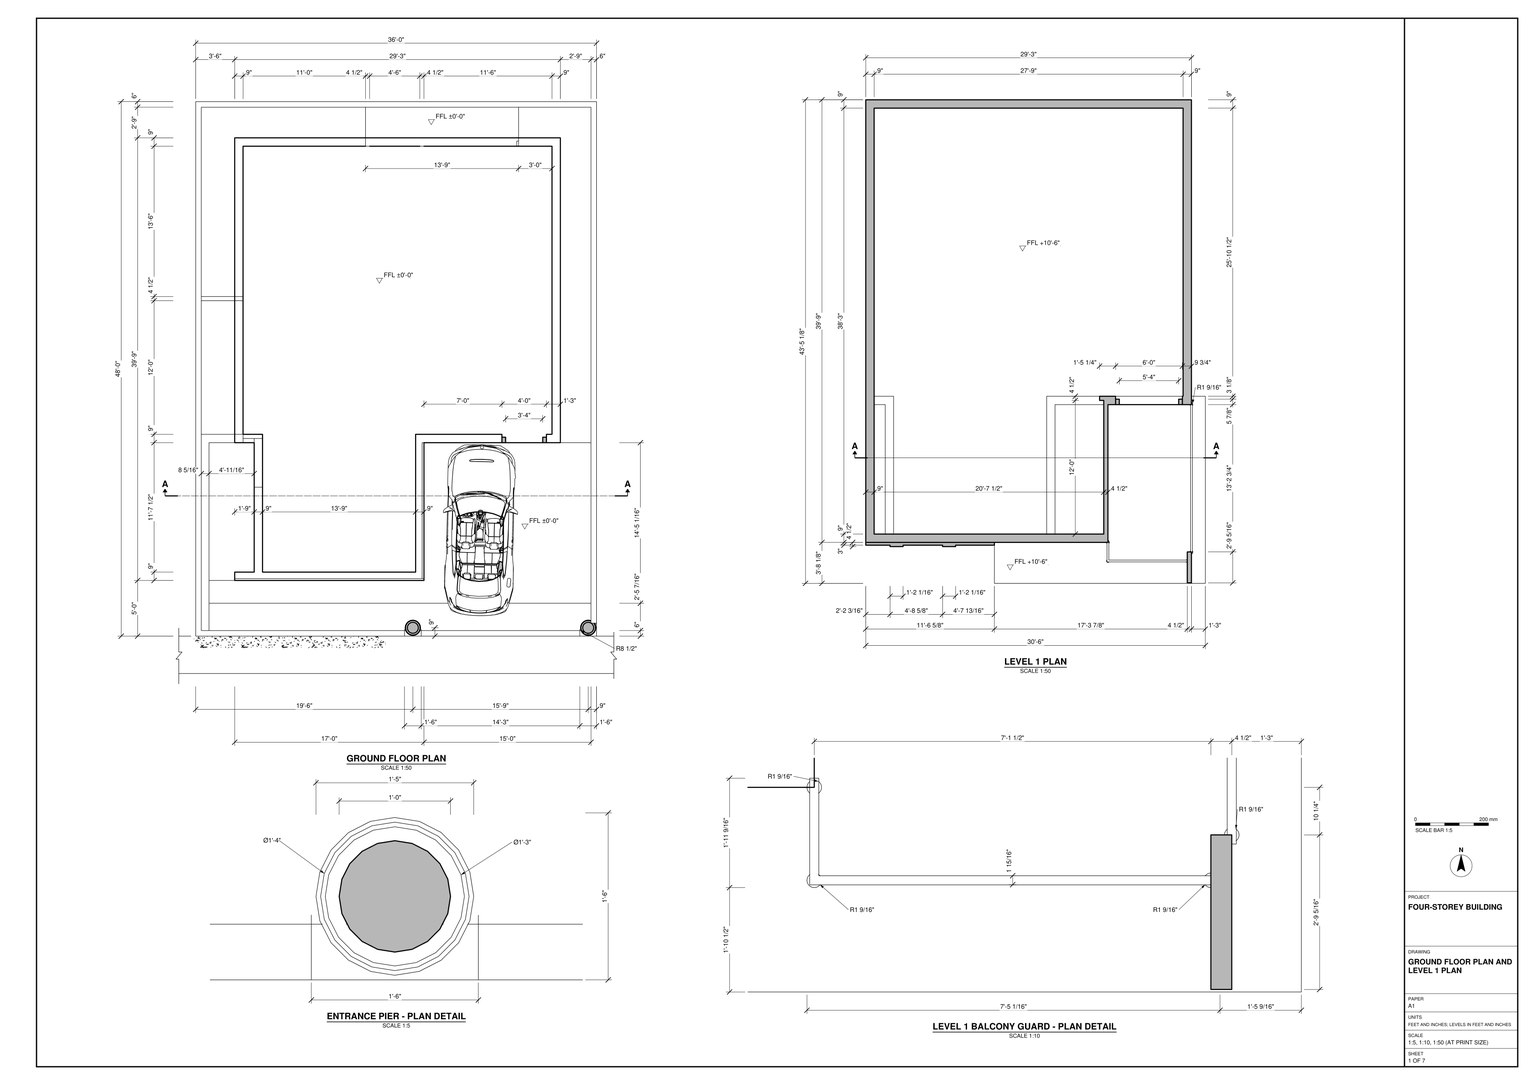
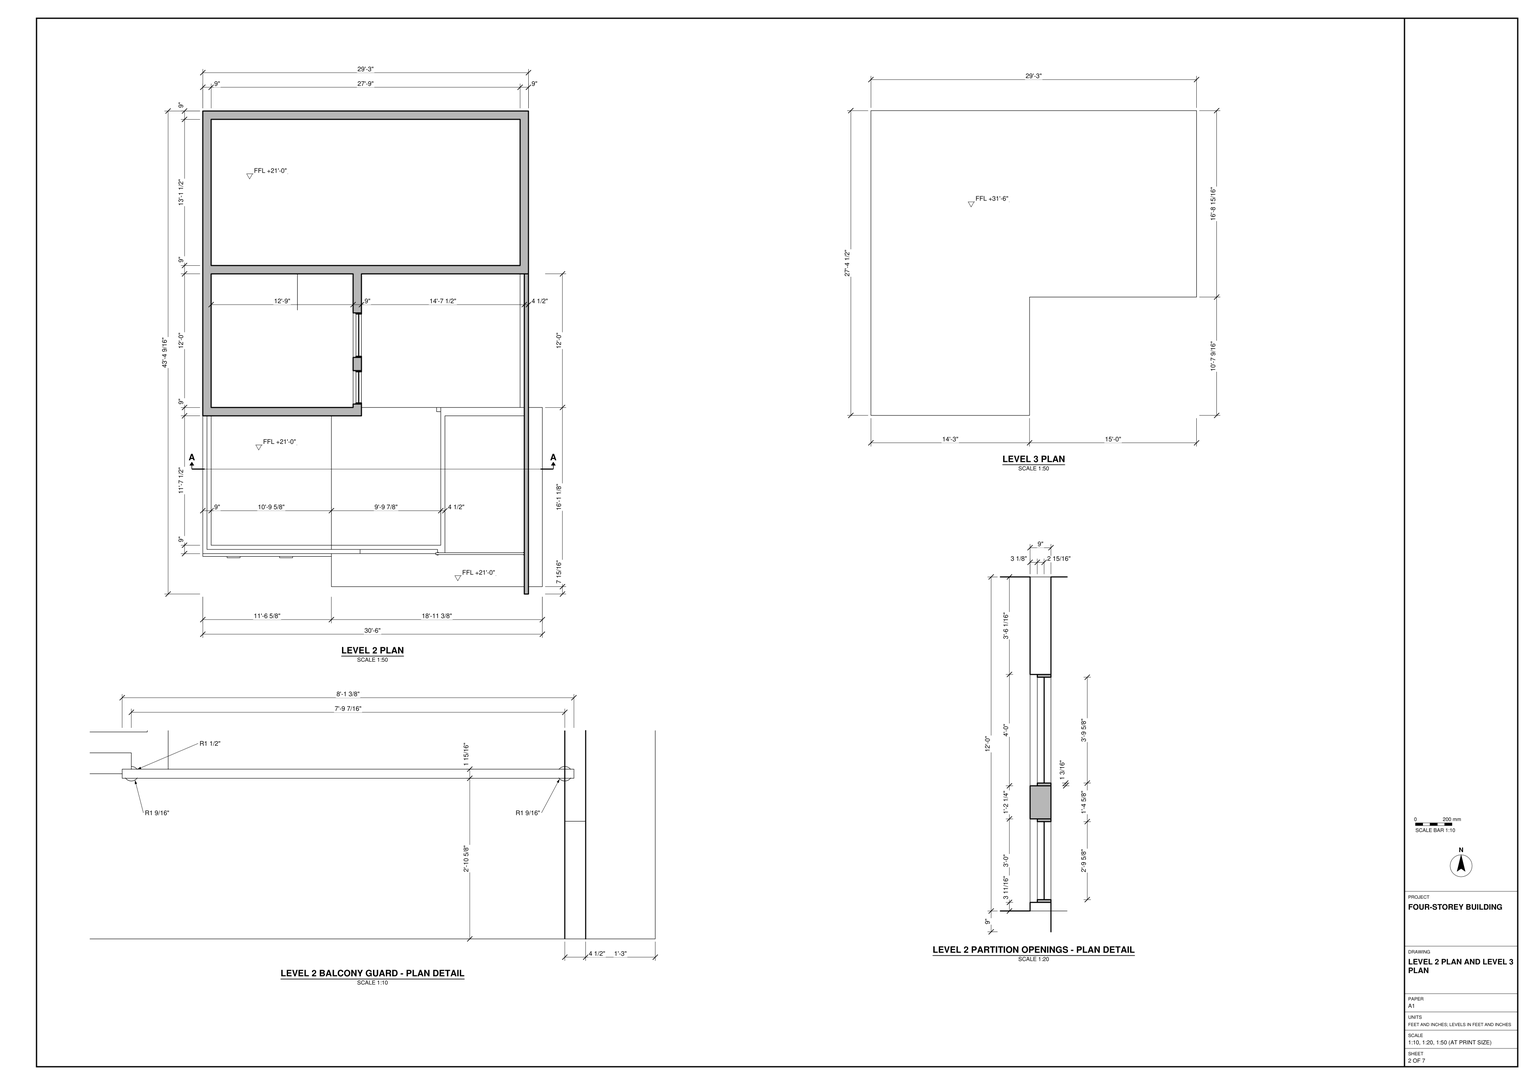
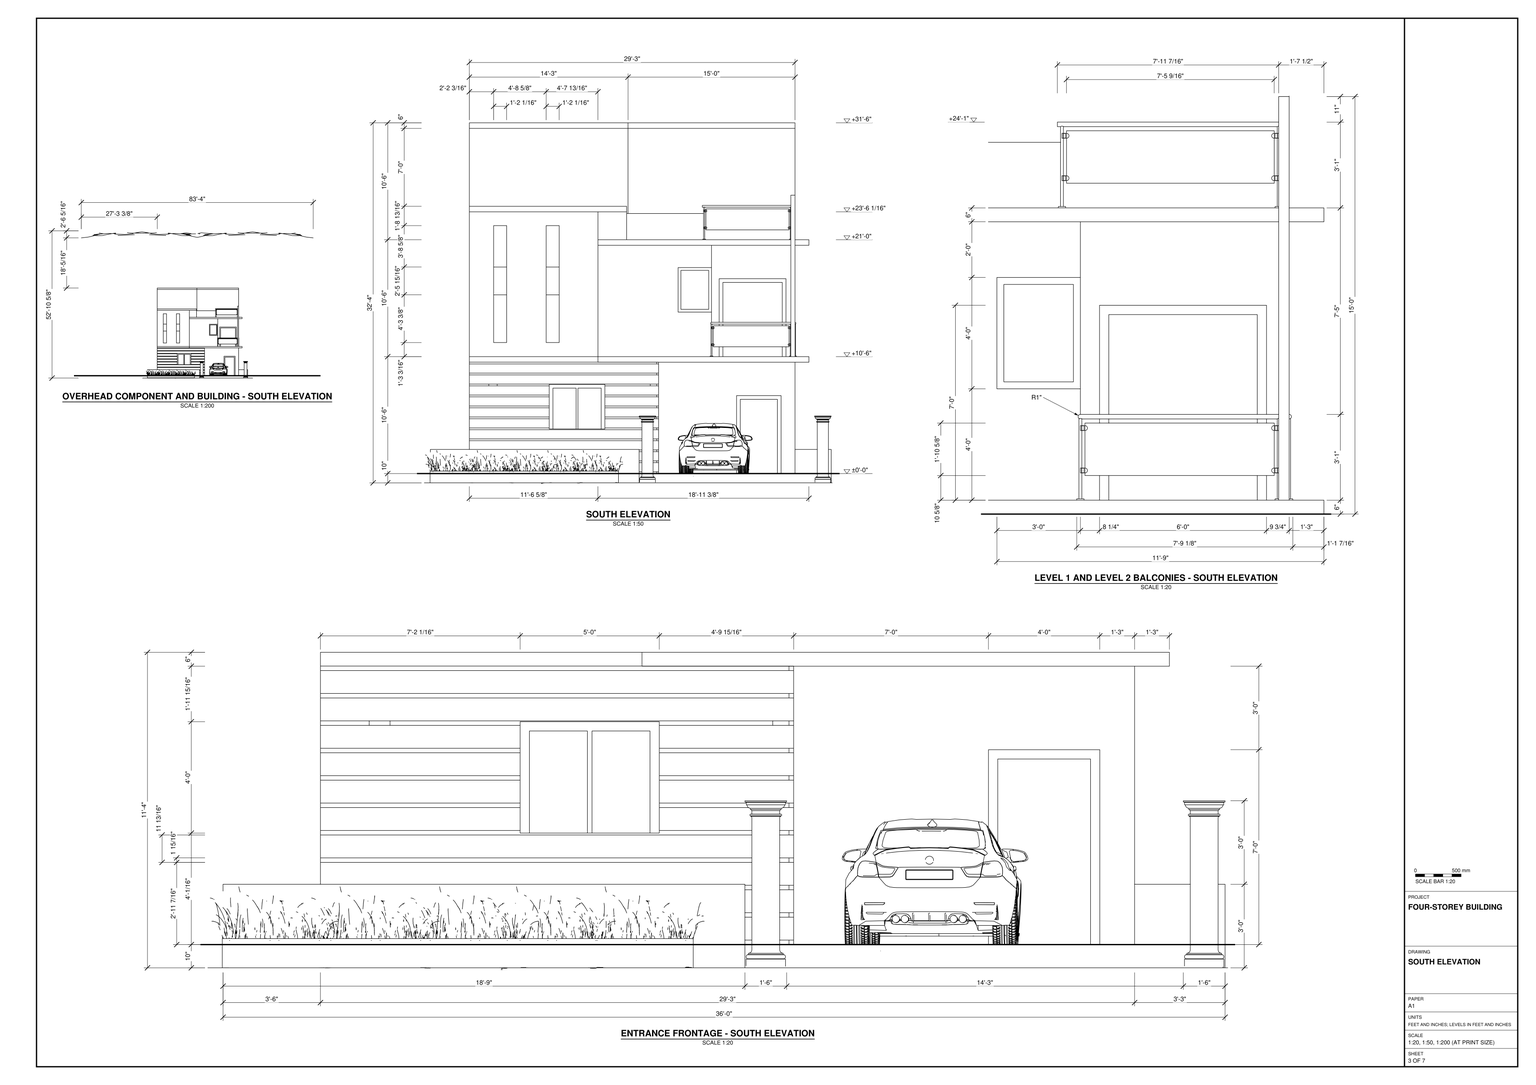
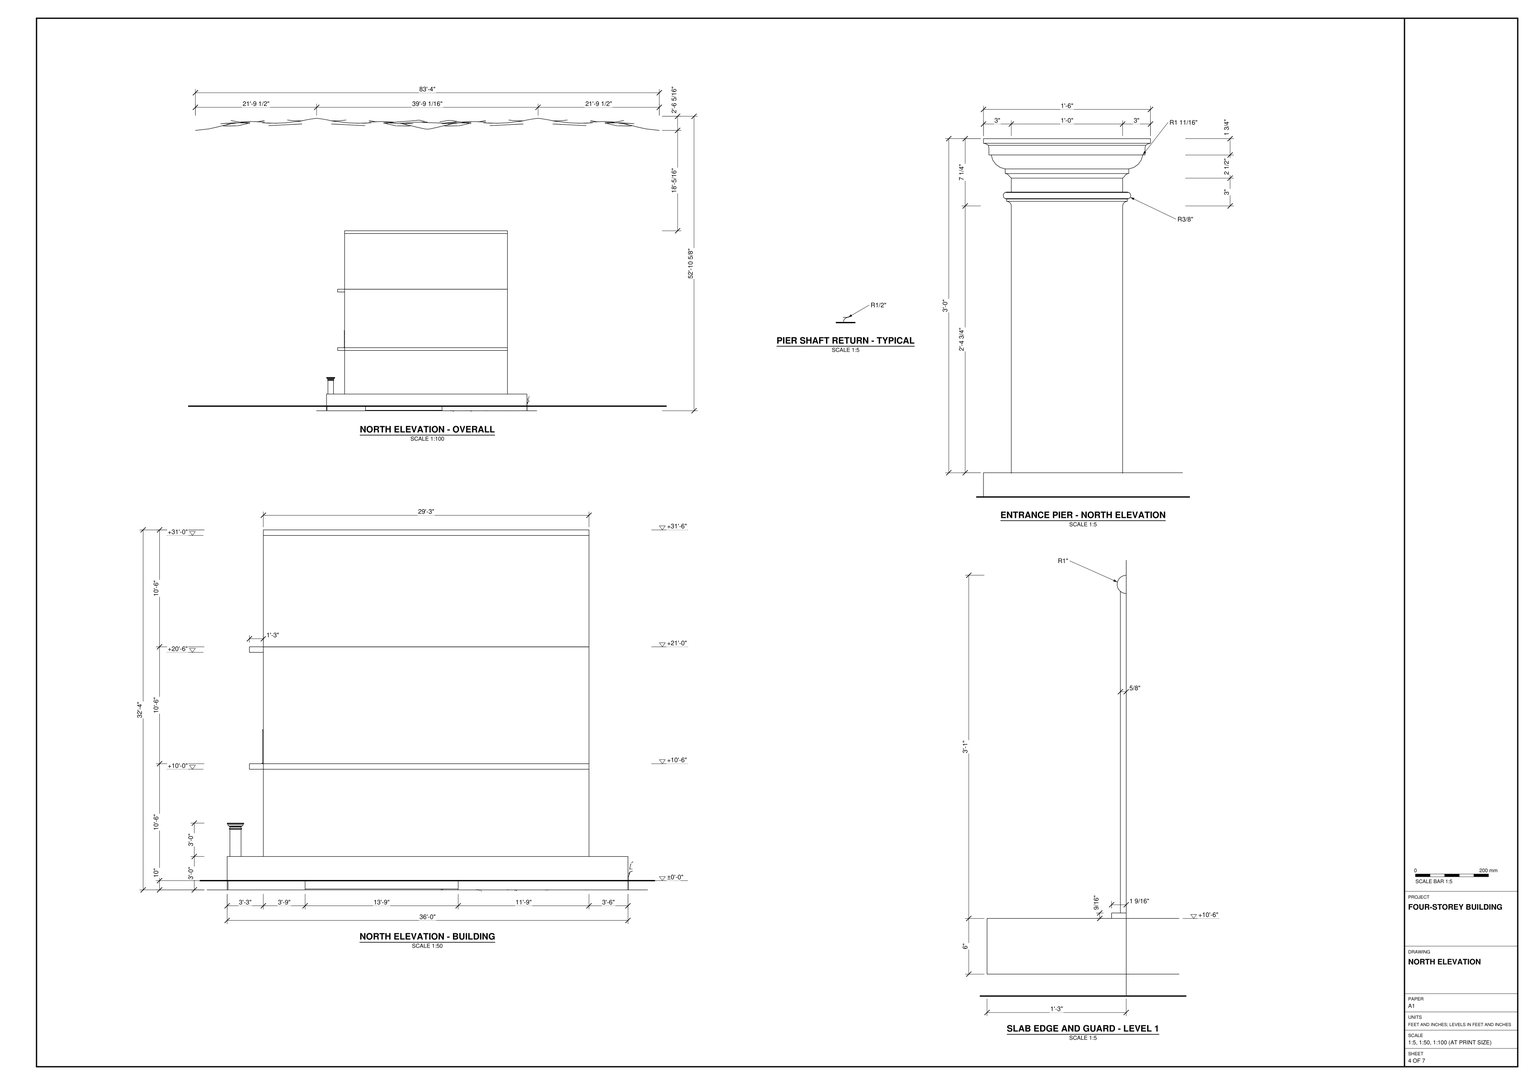
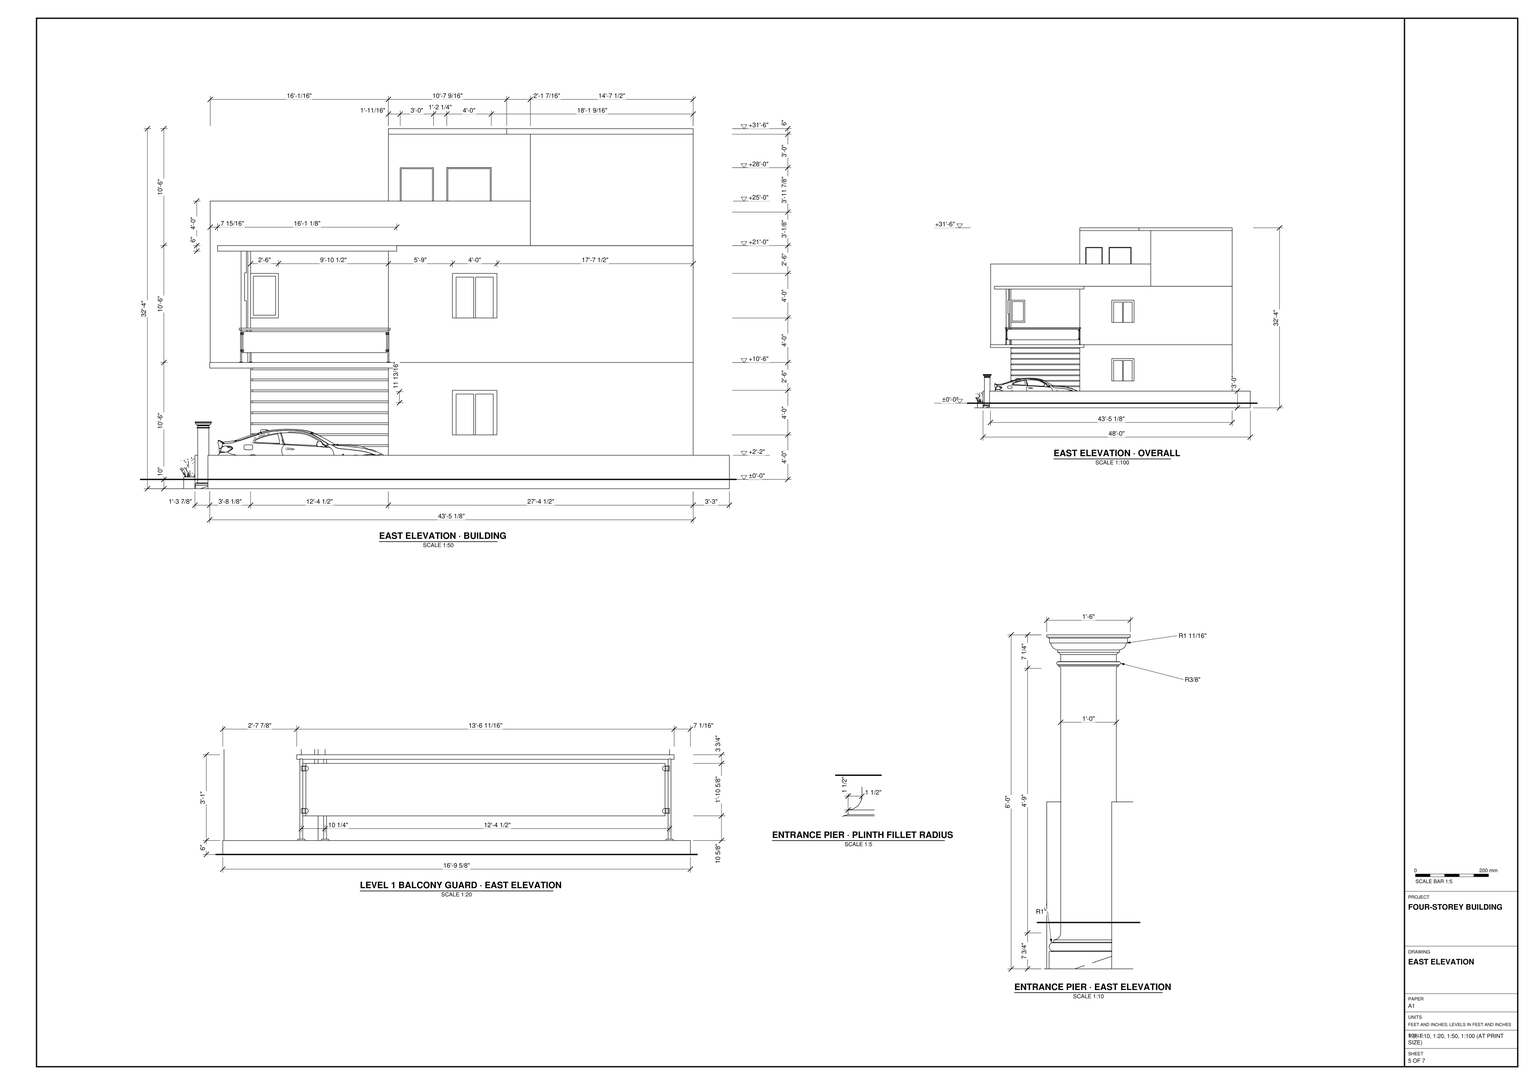
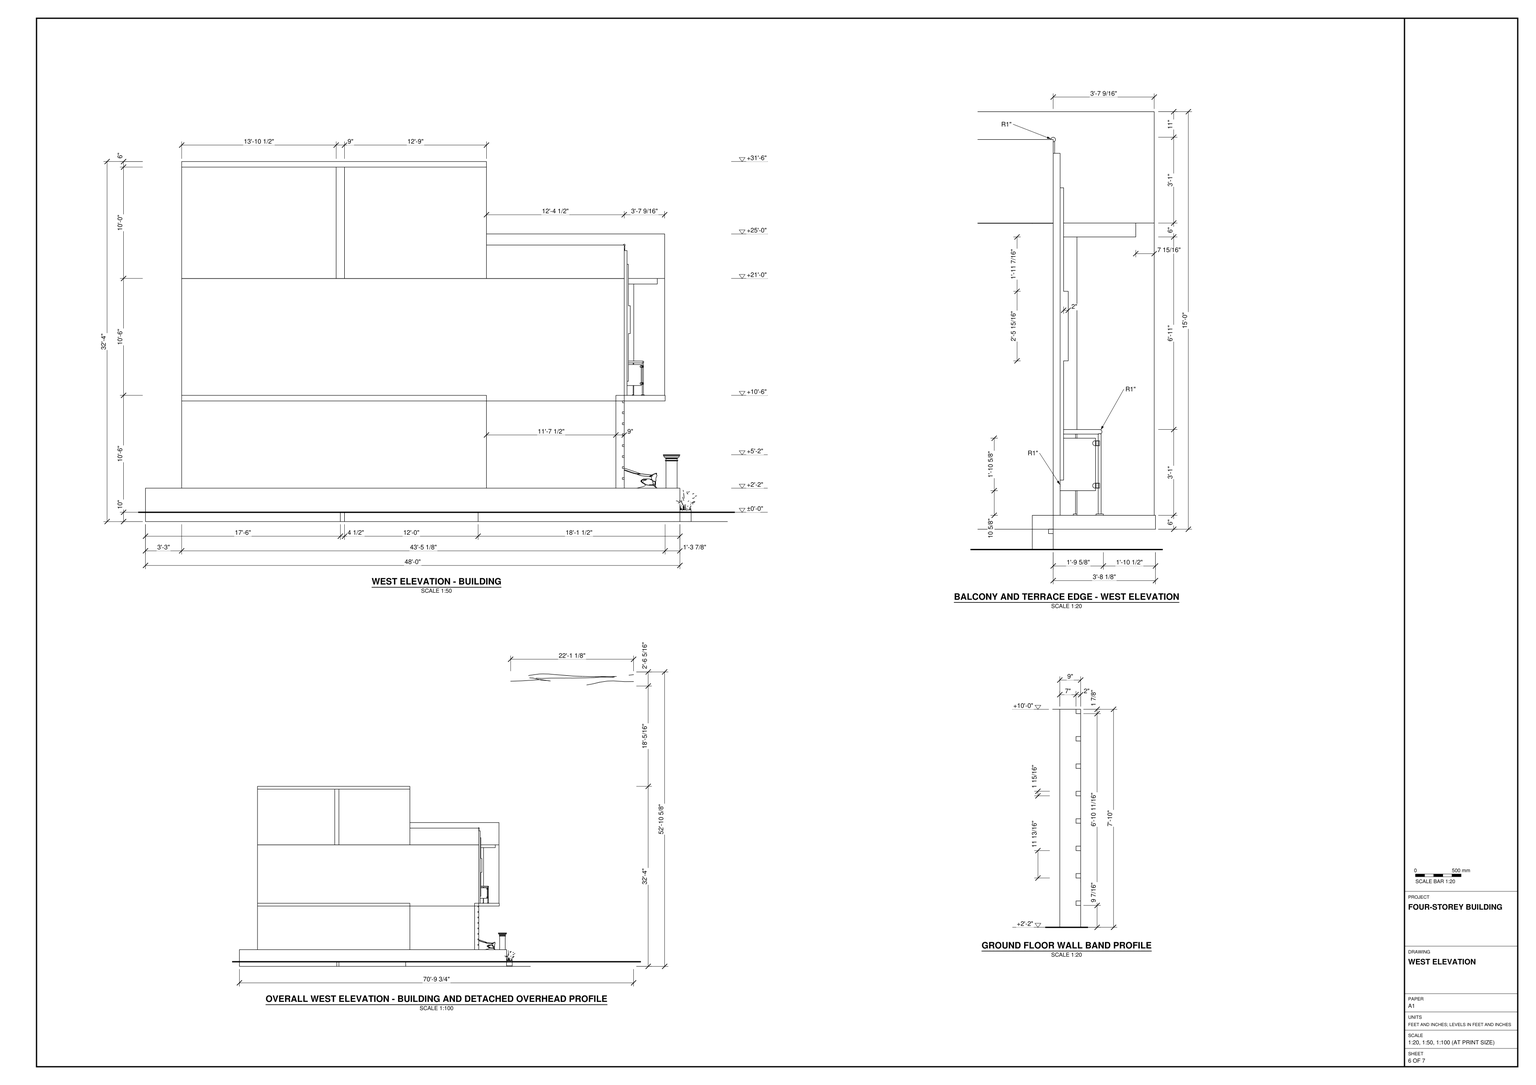
Build the four-storey building and its site in SketchUp using task_files/diagram_01.pdf. Work in feet and inches. The complete model, including the overhead element shown in the small south elevation, measures 83'-4" along X, 70'-9 3/4" along Y and 52'-10 5/8" along Z. Use the ground floor at ±0'-0" as the datum and set the successive levels at +10'-6", +21'-0" and +31'-6".

Lay out the site and the stepped ground-floor footprint from the plan. Leave the entrance and parking recess on the right as seen from the south. Place the entrance piers on either side of the drive and the planting strip to its left. Match the wall thicknesses indicated on the plans, including the 9" walls and the thinner 4 1/2" wall sections. Follow each floor outline separately: the balcony slabs project beyond the enclosed walls, and the flat roof has an L-shaped outline. Use the plan details and south elevation together to locate the balcony guards, the framed openings and the openings in the Level 2 partition. Reproduce the horizontal bands around the ground-floor front window and the tall narrow strips above them.

Keep shell elements such as walls, slabs and roof, and each furniture or joinery piece shown, in separate groups or components; use components for repeated parts. Decor and loose items, including the planting and parked car, may be any suitable library components. Save one SketchUp model as output_files/four_storey_building_with_balconies_and_entrance_court.skp.

# SketchUp Ruby script. Lengths in inches.
U = 1.inch
M = Sketchup.active_model
def pt(a) = Geom::Point3d.new(a.map { |v| v * U })
def face(e, loops, mat)
  f = e.add_face(loops[0].map { |a| pt(a) })
  loops[1..].each { |l| e.add_face(l.map { |a| pt(a) }).erase! }
  f.material = f.back_material = mat if mat
  f
end
# faces: each face lists its corners as indices into pts; further lists are holes
def faces(e, pts, list, mat = nil) = list.each { |f| face(e, (f[0].is_a?(Array) ? f : [f]).map { |l| l.map { |i| pts[i] } }, mat) }
# xy, xz, yz: faces in a plane at the given z, y or x. An outline is a flat list of corners, or four numbers for a rectangle; further outlines are holes
def ring(l) = l.size == 4 ? [[l[0], l[1]], [l[2], l[1]], [l[2], l[3]], [l[0], l[3]]] : l.each_slice(2).to_a
def flat(e, list, mat, &to3) = list.each { |f| face(e, (f[0].is_a?(Array) ? f : [f]).map { |l| ring(l).map { |u, v| to3.(u, v) } }, mat) }
def xy(e, z, list, mat = nil) = flat(e, list, mat) { |x, y| [x, y, z] }
def xz(e, y, list, mat = nil) = flat(e, list, mat) { |x, z| [x, y, z] }
def yz(e, x, list, mat = nil) = flat(e, list, mat) { |y, z| [x, y, z] }
def lines(e, pts, list) = list.each { |a, b| e.add_line(pt(pts[a]), pt(pts[b])) }
# prism: a flat outline (further loops are holes) pulled along v
def prism(e, loops, v, mat = nil)
  f = face(e, loops, mat); d = Geom::Vector3d.new(v.map { |x| x * U })
  f.pushpull(f.normal.samedirection?(d) ? d.length : -d.length)
end
def box(e, o, s, mat = nil) = prism(e, [[o, [o[0] + s[0], o[1], o[2]], [o[0] + s[0], o[1] + s[1], o[2]], [o[0], o[1] + s[1], o[2]]]], [0, 0, s[2]], mat)
def at(x, y, z, deg = 0) = Geom::Transformation.translation(pt([x, y, z])) * Geom::Transformation.rotation(ORIGIN, Z_AXIS, deg.degrees)
def axes(o, x, y, z) = Geom::Transformation.new([*x, 0, *y, 0, *z, 0, *pt(o).to_a, 1])
def part(name) = M.definitions.add(name)
# library, detail: a bought-in or finely detailed component or shape, given as its bounding box
def library(name, o, s) = part(name).tap { |d| box(d.entities, o, s) }
def detail(e, o, s) = box(e.add_group.entities, o, s)
def put(e, d, t, mat = nil) = e.add_instance(d, t).tap { |i| i.material = mat if mat }
def group(e, t, mat = nil) = e.add_group.tap { |g| g.transformation = t; g.material = mat if mat }.entities
root = M.entities
M.materials.add("[Color C06]").color = [204, 102, 0]
M.materials.add("[Color C07]").color = [153, 76, 0]
M.materials.add("[Color C08]").color = [102, 51, 0]
M.materials.add("[Color D01]").color = [255, 242, 204]
M.materials.add("[Color I03]").color = [101, 101, 255]
M.materials.add("[Color M06]").color = [86, 86, 86]
M.materials.add("[Color M07]").color = [58, 58, 58]
M.materials.add("[Tile Ceramic Natural]").color = [189, 180, 134]
M.materials.add("[Translucent Glass Blue]").color = [100, 149, 237]
M.materials.add("[Wood Cherry Original]").color = [152, 86, 42]
M.materials.add("[Wood Veneer 01]").color = [120, 70, 37]
M.materials.add("[Wood Veneer 02]").color = [190, 128, 91]
c1 = part("new bloSDFck")
p = [[-0.99,-2.25,0],[-22.01,-2.25,0],[-0.99,-4.5,0],[-0.99,0,0],[0.99,0,0],[0.99,-4.5,0],
  [-24,-4.5,0],[-24,0,0],[-22.01,0,0],[-22.01,-4.5,0],[22.01,-4.5,0],[22.01,0,0],
  [24,0,0],[24,-4.5,0],[24,4.5,0],[-24,4.5,0],[22.01,-2.25,0],[0.99,-2.25,0]]
lines(c1.entities,p,[[0,1],[2,3],[4,5],[6,7],[7,8],[8,9],[10,11],[11,12],[12,13],[13,6],[13,14],[6,15],
  [15,14],[12,7],[16,17]])
c2 = part("A$C63CB6BFC")
p = [[-24,-4.5,0],[24,-4.5,0],[24,0,0],[-24,0,0],[22.01,2.25,0],[1.02,2.25,0],
  [-0.96,2.25,0],[-22.01,2.25,0],[-0.96,4.5,0],[-0.96,0,0],[1.02,0,0],[1.02,4.5,0],
  [-22.01,0,0],[-22.01,4.5,0],[22.01,0,0],[24,4.5,0],[-24,4.5,0],[22.01,4.5,0]]
lines(c2.entities,p,[[0,1],[2,3],[4,5],[6,7],[8,9],[9,10],[10,11],[3,12],[12,13],[14,2],[15,16],[15,1],
  [16,0],[17,14]])
c3 = part("A$C1F62275E")
p = [[30,-4.5,0],[-30,-4.5,0],[-30,0,0],[30,0,0],[-28.01,2.25,0],[-0.99,2.25,0],
  [0.99,2.25,0],[28.01,2.25,0],[0.99,4.5,0],[0.99,0,0],[-0.99,0,0],[-0.99,4.5,0],
  [28.01,0,0],[28.01,4.5,0],[-28.01,4.5,0],[-28.01,0,0],[-30,4.5,0],[30,4.5,0]]
lines(c3.entities,p,[[0,1],[2,3],[4,5],[6,7],[8,9],[9,10],[10,11],[3,12],[12,13],[14,15],[15,2],[16,17],
  [16,1],[17,0]])
c4 = part("VEN")
p = [[-4.5,-11.98,0],[4.5,-11.98,0],[2.25,10,0],[2.25,-10,0],[0,-11.98,0],[0,11.98,0],
  [0,-10,0],[4.5,-10,0],[4.5,10,0],[0,10,0],[4.5,11.98,0],[-4.5,11.98,0]]
lines(c4.entities,p,[[0,1],[2,3],[4,5],[6,7],[8,9],[1,10],[0,11],[10,11]])
c5 = library("002 Bmw M4 + mat3.4 2017",[-252.8,19.48,9.01],[196.94,171.32,55.15])
c6 = library("lvt__Defintion3",[-70.01,-133.44,604.33],[1000,265.15,30.32])
c7 = library("Group\#14",[0,0,0],[56.8,25.91,35.15])
c8 = library("Group\#15",[0,0,0],[56.8,25.91,35.15])
c9 = part("House+plant_11")
put(c9.entities,c6,at(96.28,168.2,0))
put(c9.entities,c7,at(305.6,289.78,0))
put(c9.entities,c7,at(349.27,289.78,0))
put(c9.entities,c8,at(392.14,289.78,0))
put(c9.entities,c7,at(425.32,289.78,0))
put(c9.entities,c7,at(463.51,289.78,0))
c10 = part("Group92\#1")
p = [[33,3,0],[3,3,0],[3,45,0],[33,45,0]]
lines(c10.entities,p,[[0,1],[1,2],[2,3],[3,0]])
c11 = part("Group93\#1")
xy(c11.entities,2.5,[[3,3,33,45]])
c12 = part("Group91\#1")
xy(c12.entities,5,[[[0,0,36,48],[3,3,33,45]]],"[Wood Veneer 01]")
xz(c12.entities,0,[[0,0,36,5]],"[Wood Veneer 01]")
xz(c12.entities,3,[[3,0,33,5]],"[Wood Veneer 01]")
xz(c12.entities,45,[[3,0,33,5]],"[Wood Veneer 01]")
xz(c12.entities,48,[[0,0,36,5]],"[Wood Veneer 01]")
yz(c12.entities,0,[[0,0,48,5]],"[Wood Veneer 01]")
yz(c12.entities,3,[[3,0,45,5]],"[Wood Veneer 01]")
yz(c12.entities,33,[[3,0,45,5]],"[Wood Veneer 01]")
put(c12.entities,c10,at(0,0,0))
put(c12.entities,c11,at(0,0,0),"[Translucent Glass Blue]")
c13 = part("Group95\#1")
p = [[3,-45,0],[3,-3,0],[27,-3,0],[27,-45,0]]
lines(c13.entities,p,[[0,1],[1,2],[2,3],[3,0]])
c14 = part("Group96\#1")
xy(c14.entities,2.5,[[3,-45,27,-3]])
c15 = part("Group94\#1")
xy(c15.entities,5,[[[0,-48,30,0],[3,-45,27,-3]]],"[Wood Veneer 01]")
xz(c15.entities,-48,[[0,0,30,5]],"[Wood Veneer 01]")
xz(c15.entities,-45,[[3,0,27,5]],"[Wood Veneer 01]")
xz(c15.entities,-3,[[3,0,27,5]],"[Wood Veneer 01]")
xz(c15.entities,0,[[0,0,30,5]],"[Wood Veneer 01]")
yz(c15.entities,3,[[-45,0,-3,5]],"[Wood Veneer 01]")
yz(c15.entities,27,[[-45,0,-3,5]],"[Wood Veneer 01]")
yz(c15.entities,30,[[-48,0,0,5]],"[Wood Veneer 01]")
put(c15.entities,c13,at(0,0,0))
put(c15.entities,c14,at(0,0,0),"[Translucent Glass Blue]")
c16 = library("Group\#6",[-56.375,-20.6,0],[227.375,193.1,6])
c17 = part("Group99\#2")
xy(c17.entities,0,[[0,0,19,44]])
c18 = part("Group97\#1")
xy(c18.entities,0,[[0,0,0,48,48,48,48,0,44,0,44,44,25,44,25,0,23,0,23,44,4,44,4,0]])
xy(c18.entities,4,[[0,0,4,0,4,44,23,44,23,0,25,0,25,44,44,44,44,0,48,0,48,48,0,48]],"[Wood Veneer 01]")
xz(c18.entities,0,[[0,0,4,4],[23,0,25,4],[44,0,48,4]])
xz(c18.entities,44,[[4,0,23,4],[25,0,44,4]])
xz(c18.entities,48,[[0,0,48,4]])
yz(c18.entities,0,[[0,0,48,4]])
yz(c18.entities,4,[[0,0,44,4]])
yz(c18.entities,23,[[0,0,44,4]])
yz(c18.entities,25,[[0,0,44,4]])
yz(c18.entities,44,[[0,0,44,4]])
yz(c18.entities,48,[[0,0,48,4]])
# 3 loose lines left out
put(c18.entities,c17,at(4,0,2))
put(c18.entities,c17,at(25,0,2))
c19 = part("Group103\#1")
xy(c19.entities,0,[[-36,-42,-36,42,36,42,36,-42,32,-42,32,38,-32,38,-32,-42]])
xy(c19.entities,5.875,[[-36,-42,-32,-42,-32,38,32,38,32,-42,36,-42,36,42,-36,42]],"[Wood Veneer 01]")
xz(c19.entities,-42,[[-36,0,-32,5.875],[32,0,36,5.875]])
xz(c19.entities,38,[[-32,0,32,5.875]])
xz(c19.entities,42,[[-36,0,36,5.875]])
yz(c19.entities,-36,[[-42,0,42,5.875]])
yz(c19.entities,-32,[[-42,0,38,5.875]])
yz(c19.entities,32,[[-42,0,38,5.875]])
yz(c19.entities,36,[[-42,0,42,5.875]])
c20 = part("Difference")
xy(c20.entities,0,[[9,9,256.5,9,256.5,153,252,153,252,157.5,269.25,157.5,269.25,148.5,341.25,148.5,341.25,157.5,342,157.5,342,468,9,468]])
xy(c20.entities,48,[[225,0,261,0,261,30,256.5,30,256.5,9,225,9],[342,217.5,351,265.5]])
xy(c20.entities,84,[[269.25,148.5,341.25,157.5]])
xy(c20.entities,96,[[225,0,225,9,256.5,9,256.5,30,261,30,261,0],[342,217.5,351,265.5]])
xy(c20.entities,125.875,[[[0,0,261,0,261,148.5,351,148.5,351,477,0,477],[9,9,9,468,342,468,342,157.5,252,157.5,252,153,256.5,153,256.5,9]]])
xz(c20.entities,0,[[0,0,138.625,125.875]])
xz(c20.entities,0,[[138.625,0,261,0,261,48,225,48,225,96,261,96,261,125.875,138.625,125.875]],"[Wood Veneer 02]")
xz(c20.entities,9,[[9,0,9,125.875,256.5,125.875,256.5,96,225,96,225,48,256.5,48,256.5,0]])
xz(c20.entities,30,[[256.5,48,261,96]])
xz(c20.entities,148.5,[[261,-6,269.25,-6,269.25,84,341.25,84,341.25,-6,351,-6,351,125.875,261,125.875],[269.25,-6,341.25,0]])
xz(c20.entities,153,[[252,-6,256.5,0],[252,0,256.5,125.875]])
xz(c20.entities,157.5,[[252,-6,269.25,0],[341.25,-6,342,0],[252,0,252,125.875,342,125.875,342,0,341.25,0,341.25,84,269.25,84,269.25,0]])
xz(c20.entities,217.5,[[342,48,351,96]])
xz(c20.entities,265.5,[[342,48,351,96]])
xz(c20.entities,468,[[9,-6,342,0],[9,0,342,125.875]])
xz(c20.entities,477,[[0,-6,351,125.875]])
yz(c20.entities,0,[[0,-6,477,125.875]])
yz(c20.entities,9,[[9,0,468,125.875]])
yz(c20.entities,225,[[0,48,9,96]])
yz(c20.entities,252,[[153,-6,157.5,0],[153,0,157.5,125.875]])
yz(c20.entities,256.5,[[9,0,9,48,30,48,30,96,9,96,9,125.875,153,125.875,153,0]])
yz(c20.entities,261,[[0,0,148.5,0,148.5,125.875,0,125.875,0,96,30,96,30,48,0,48]],"[Wood Veneer 02]")
yz(c20.entities,269.25,[[148.5,-6,157.5,0],[148.5,0,157.5,84]])
yz(c20.entities,341.25,[[148.5,-6,157.5,0],[148.5,0,157.5,84]])
yz(c20.entities,342,[[157.5,-6,468,0],[[157.5,0,468,125.875],[217.5,48,265.5,96]]])
yz(c20.entities,351,[[[148.5,0,477,125.875],[217.5,48,265.5,96]]])
# 5 loose lines left out
put(c20.entities,c18,axes([342,217.5,48],[0,1,0],[0,0,1],[1,0,0]))
put(c20.entities,c19,axes([305.25,154.375,42],[1,0,0],[0,0,1],[0,-1,0]))
c21 = part("Group92\#2")
xy(c21.entities,0,[[0,0,25,44]],"[Translucent Glass Blue]")
c22 = part("Group90\#1")
xy(c22.entities,0,[[0,0,0,48,60,48,60,0,56,0,56,44,31,44,31,0,29,0,29,44,4,44,4,0]])
xy(c22.entities,4,[[0,0,4,0,4,44,29,44,29,0,31,0,31,44,56,44,56,0,60,0,60,48,0,48]],"[Color M06]")
xz(c22.entities,0,[[0,0,4,4],[29,0,31,4],[56,0,60,4]])
xz(c22.entities,44,[[4,0,29,4],[31,0,56,4]])
xz(c22.entities,48,[[0,0,60,4]])
yz(c22.entities,0,[[0,0,48,4]])
yz(c22.entities,4,[[0,0,44,4]])
yz(c22.entities,29,[[0,0,44,4]])
yz(c22.entities,31,[[0,0,44,4]])
yz(c22.entities,56,[[0,0,44,4]])
yz(c22.entities,60,[[0,0,48,4]])
# 3 loose lines left out
put(c22.entities,c21,at(4,0,2))
put(c22.entities,c21,at(31,0,2))
c23 = part("Group103\#2")
xy(c23.entities,0,[[0,0,19,44]],"[Translucent Glass Blue]")
c24 = part("Group101\#1")
prism(c24.entities,[[[25,44,0],[25,0,0],[23,0,0],[23,44,0],[4,44,0],[4,0,0],[0,0,0],[0,48,0],[48,48,0],[48,0,0],[44,0,0],[44,44,0]]],[0,0,4],"[Wood Veneer 01]")
# 3 loose lines left out
put(c24.entities,c23,at(4,0,2))
put(c24.entities,c23,at(25,0,2))
c25 = part("Group104\#1")
prism(c25.entities,[[[24,42,0],[24,-42,0],[20,-42,0],[20,38,0],[-20,38,0],[-20,-42,0],[-24,-42,0],[-24,42,0]]],[0,0,5.875])
c26 = library("Group\#8",[0,0,0],[89.04,23.58,36.98])
c27 = library("Group\#9",[0,0,0],[3.15,162.6875,36.98])
c28 = part("Group120\#1")
p = [[46.8125,1.1875,0],[1.1875,1.1875,0],[1.1875,46.68,0],[46.8125,46.68,0]]
lines(c28.entities,p,[[0,1],[1,2],[2,3],[3,0]])
c29 = part("Group121\#1")
xy(c29.entities,2.9375,[[1.1875,1.1875,46.8125,46.68]],"[Translucent Glass Blue]")
c30 = part("Group119\#1")
xy(c30.entities,0,[[[0,0,48,47.87],[1.1875,1.1875,46.8125,46.68]]])
xy(c30.entities,5.875,[[[0,0,48,47.87],[1.1875,1.1875,46.8125,46.68]]],"[Wood Veneer 01]")
xz(c30.entities,0,[[0,0,48,5.875]])
xz(c30.entities,1.1875,[[1.1875,0,46.8125,5.875]],"[Wood Veneer 01]")
xz(c30.entities,46.68,[[1.1875,0,46.8125,5.875]])
xz(c30.entities,47.87,[[0,0,48,5.875]])
yz(c30.entities,0,[[0,0,47.87,5.875]])
yz(c30.entities,1.1875,[[1.1875,0,46.68,5.875]])
yz(c30.entities,46.8125,[[1.1875,0,46.68,5.875]],"[Wood Veneer 01]")
yz(c30.entities,48,[[0,0,47.87,5.875]])
put(c30.entities,c28,at(0,0,0))
put(c30.entities,c29,at(0,0,0))
c31 = part("Group117\#1")
p = [[-1.1875,82.8125,0],[-1.1875,1.1875,0],[-34.8125,1.1875,0],[-34.8125,82.8125,0]]
lines(c31.entities,p,[[0,1],[1,2],[2,3],[3,0]])
c32 = part("Group118\#1")
xy(c32.entities,2.9375,[[-34.8125,1.1875,-1.1875,82.8125]])
c33 = part("Group116\#1")
prism(c33.entities,[[[-36,84,0],[0,84,0],[0,0,0],[-36,0,0]],[[-1.1875,1.1875,0],[-1.1875,82.8125,0],[-34.8125,82.8125,0],[-34.8125,1.1875,0]]],[0,0,5.875])
put(c33.entities,c31,at(0,0,0))
put(c33.entities,c32,at(0,0,0))
c34 = library("Group172\#1",[8097.16,1237.06,0],[18,18,72])
c35 = library("Group\#10",[0,0,0],[97.38,3.15,36.98])
xy(root,10,[[14.3125,35.45,426,35.45,426,208.5,246,208.5,246,60,14.3125,60]],"[Tile Ceramic Natural]")
xy(root,136,[[388.5,16.4375,393,49.75],[42,57,180.625,60]])
xy(root,151.2,[[68.16,55.5,82.23,57],[124.79,55.5,138.85,57]])
xy(root,202.6,[[68.16,53.5,82.23,55.5],[124.79,53.5,138.85,55.5]])
xy(root,232.56,[[68.16,53.5,82.23,55.5],[124.79,53.5,138.85,55.5]])
xy(root,277.2,[[68.16,55.5,82.23,57],[124.79,55.5,138.85,57]])
xy(root,292.05,[[42,57,180.625,60]])
xz(root,16.4375,[[388.5,136,393,310]],"[Color D01]")
xz(root,49.75,[[388.5,136,393,262]],"[Color D01]")
xz(root,53.5,[[68.16,202.6,82.23,232.56],[124.79,202.6,138.85,232.56]],"[Color I03]")
xz(root,55.5,[[68.16,151.2,82.23,202.6],[124.79,151.2,138.85,202.6],[68.16,232.56,82.23,277.2],[124.79,232.56,138.85,277.2]],"[Color D01]")
xz(root,57,[[[42,136,180.625,292.05],[68.16,151.2,82.23,277.2],[124.79,151.2,138.85,277.2]]])
xz(root,60,[[42,136,180.625,292.05]])
xz(root,208.5,[[334,10,374,90]],"[Wood Cherry Original]")
yz(root,42,[[57,136,60,292.05]])
yz(root,68.16,[[55.5,151.2,55.5,202.6,53.5,202.6,53.5,232.56,55.5,232.56,55.5,277.2,57,277.2,57,151.2]])
yz(root,82.23,[[55.5,151.2,57,151.2,57,277.2,55.5,277.2,55.5,232.56,53.5,232.56,53.5,202.6,55.5,202.6]],"[Color I03]")
yz(root,124.79,[[55.5,151.2,55.5,202.6,53.5,202.6,53.5,232.56,55.5,232.56,55.5,277.2,57,277.2,57,151.2]])
yz(root,138.85,[[55.5,151.2,57,151.2,57,277.2,55.5,277.2,55.5,232.56,53.5,232.56,53.5,202.6,55.5,202.6]],"[Color I03]")
yz(root,180.625,[[57,136,60,292.05]])
yz(root,388.5,[[16.4375,262,361.5,310]])
yz(root,388.5,[[16.4375,136,49.75,262]],"[Color D01]")
yz(root,393,[[16.4375,136,49.75,136,49.75,262,361.5,262,361.5,310,16.4375,310]],"[Color D01]")
# 100 loose lines left out
put(root,c1,at(46.5,289.5,10,90))
put(root,c2,axes([144,532.5,10],[1,0,0],[0,-1,0],[0,0,1]))
put(root,c3,at(158,64.5,10))
put(root,c4,at(214.58,532.5,10,-90))
put(root,c5,at(130.44,52.04,0,-126.296))
put(root,c9,at(-311.65,-308.5,0),"[Color C07]")
put(root,c12,axes([267,65,184],[1,0,0],[0,0,1],[0,-1,0]))
put(root,c15,axes([298,60,232],[0,1,0],[0,0,1],[1,0,0]))
g1 = group(root,at(315.25,208.5,136))
xz(g1,0,[[0,0,64,80]],"[Translucent Glass Blue]")
g2 = group(root,at(-709.92,-151.5625,146.75))
prism(g2,[[[1008.42,369.0625,109.25],[1008.42,220.5625,109.25],[760.92,220.5625,109.25],[760.92,679.5625,109.25],[1093.92,679.5625,109.25],[1093.92,369.0625,109.25]]],[0,0,6])
put(root,c16,at(237,45,256),"[Color D01]")
put(root,c20,at(42,60,136),"[Color D01]")
g3 = group(root,at(-18.27,-51.32,10),"[Color D01]")
xy(g3,0,[[396.27,259.82,396.27,268.82,402.27,268.82,402.27,579.32,366.27,579.32,366.27,588.32,411.27,588.32,411.27,259.82],[364.27,579.32,366.27,584.82]])
xy(g3,0,[[60.27,111.32,264.27,113.32],[60.27,113.32,60.27,120.32,81.27,120.32,81.27,211.82,90.27,211.82,90.27,120.32,255.27,120.32,255.27,268.82,348.27,268.82,348.27,259.82,262.27,259.82,262.27,113.32],[262.27,113.32,264.27,259.82]],"[Color C06]")
xy(g3,1.9375,[[262.27,113.32,264.27,259.82]])
xy(g3,1.9375,[[60.27,111.32,262.27,113.32],[262.27,111.32,264.27,113.32]],"[Color C06]")
xy(g3,11.8125,[[60.27,111.32,262.27,113.32],[262.27,111.32,264.27,113.32],[262.27,113.32,264.27,259.82]],"[Color C06]")
xy(g3,13.75,[[60.27,111.32,262.27,113.32],[262.27,111.32,264.27,113.32],[262.27,113.32,264.27,259.82]])
xy(g3,23.625,[[60.27,111.32,262.27,113.32],[262.27,111.32,264.27,113.32],[262.27,113.32,264.27,259.82]],"[Color C06]")
xy(g3,25.5625,[[262.27,113.32,264.27,259.82]])
xy(g3,25.5625,[[60.27,111.32,262.27,113.32],[262.27,111.32,264.27,113.32]],"[Color C06]")
xy(g3,35.4375,[[60.27,111.32,262.27,113.32],[262.27,111.32,264.27,113.32],[262.27,113.32,264.27,259.82]],"[Color C06]")
xy(g3,37.375,[[60.27,111.32,262.27,113.32],[262.27,111.32,264.27,113.32],[262.27,113.32,264.27,259.82]])
xy(g3,47.25,[[262.27,113.32,264.27,259.82]],"[Color C06]")
xy(g3,47.25,[[60.27,111.32,262.27,113.32],[262.27,111.32,264.27,113.32]],"[Color C08]")
xy(g3,48,[[402.27,328.82,411.27,376.82]])
xy(g3,48.08,[[146.35,111.32,206.35,113.32],[146.35,113.32,206.35,120.32]])
xy(g3,49.1875,[[60.27,111.32,146.35,113.32],[262.27,113.32,264.27,259.82]])
xy(g3,49.1875,[[206.35,111.32,262.27,113.32],[262.27,111.32,264.27,113.32]],"[Color C06]")
xy(g3,59.0625,[[60.27,111.32,146.35,113.32]])
xy(g3,59.0625,[[262.27,113.32,264.27,259.82]],"[Color C06]")
xy(g3,59.0625,[[206.35,111.32,262.27,113.32],[262.27,111.32,264.27,113.32]],"[Color C08]")
xy(g3,61,[[60.27,111.32,146.35,113.32],[262.27,113.32,264.27,259.82]])
xy(g3,61,[[206.35,111.32,262.27,113.32],[262.27,111.32,264.27,113.32]],"[Color C06]")
xy(g3,70.875,[[60.27,111.32,146.35,113.32]])
xy(g3,70.875,[[262.27,113.32,264.27,259.82]],"[Color C06]")
xy(g3,70.875,[[206.35,111.32,262.27,113.32],[262.27,111.32,264.27,113.32]],"[Color C08]")
xy(g3,72.8125,[[60.27,111.32,146.35,113.32],[206.35,111.32,262.27,113.32],[262.27,111.32,264.27,113.32],[262.27,113.32,264.27,259.82]])
xy(g3,82.6875,[[60.27,111.32,146.35,113.32]])
xy(g3,82.6875,[[262.27,113.32,264.27,259.82]],"[Color C06]")
xy(g3,82.6875,[[206.35,111.32,262.27,113.32],[262.27,111.32,264.27,113.32]],"[Color C08]")
xy(g3,84,[[348.27,259.82,396.27,268.82]])
xy(g3,84.625,[[60.27,111.32,146.35,113.32],[206.35,111.32,262.27,113.32],[262.27,111.32,264.27,113.32],[262.27,113.32,264.27,259.82]])
xy(g3,94.5,[[60.27,111.32,146.35,113.32]])
xy(g3,94.5,[[262.27,113.32,264.27,259.82]],"[Color C06]")
xy(g3,94.5,[[206.35,111.32,262.27,113.32],[262.27,111.32,264.27,113.32]],"[Color C08]")
xy(g3,96,[[402.27,328.82,411.27,376.82]])
xy(g3,96.08,[[146.35,111.32,206.35,120.32]])
xy(g3,96.4375,[[262.27,113.32,264.27,259.82]])
xy(g3,96.4375,[[60.27,111.32,262.27,113.32],[262.27,111.32,264.27,113.32]],"[Color C06]")
xy(g3,106.3125,[[262.27,113.32,264.27,259.82]],"[Color C06]")
xy(g3,106.3125,[[60.27,111.32,262.27,113.32],[262.27,111.32,264.27,113.32]],"[Color C08]")
xy(g3,108.25,[[60.27,111.32,262.27,113.32],[262.27,111.32,264.27,113.32],[262.27,113.32,264.27,259.82]])
xy(g3,118.125,[[262.27,113.32,264.27,259.82]],"[Color C06]")
xy(g3,118.125,[[60.27,111.32,262.27,113.32],[262.27,111.32,264.27,113.32]],"[Color C08]")
xy(g3,120.0625,[[262.27,113.32,264.27,259.82]],"[Color C06]")
xy(g3,120.0625,[[60.27,111.32,262.27,113.32],[262.27,111.32,264.27,113.32]],"[Color C08]")
xy(g3,126,[[60.27,111.32,264.27,111.32,264.27,259.82,411.27,259.82,411.27,588.32,60.27,588.32,60.27,259.82,81.27,259.82,81.27,120.32,60.27,120.32]])
xz(g3,111.32,[[60.27,1.9375,264.27,11.8125],[60.27,13.75,264.27,23.625],[60.27,25.5625,264.27,35.4375],[60.27,37.375,264.27,47.25],[60.27,49.1875,146.35,59.0625],
  [206.35,49.1875,264.27,59.0625],[60.27,61,146.35,70.875],[206.35,61,264.27,70.875],[60.27,72.8125,146.35,82.6875],[206.35,72.8125,264.27,82.6875],
  [60.27,84.625,146.35,94.5],[206.35,84.625,264.27,94.5],[60.27,96.4375,264.27,106.3125],[60.27,108.25,264.27,118.125],[60.27,120.0625,264.27,126]],"[Color C07]")
xz(g3,113.32,[[60.27,0,262.27,1.9375],[262.27,0,264.27,1.9375],[60.27,11.8125,262.27,13.75],[262.27,11.8125,264.27,13.75],[60.27,23.625,262.27,25.5625],
  [262.27,23.625,264.27,25.5625],[60.27,35.4375,262.27,37.375],[262.27,35.4375,264.27,37.375],[60.27,47.25,262.27,47.25,262.27,49.1875,206.35,49.1875,206.35,48.08,146.35,48.08,146.35,49.1875,60.27,49.1875],[262.27,47.25,264.27,49.1875],
  [60.27,59.0625,146.35,61],[206.35,59.0625,262.27,61],[262.27,59.0625,264.27,61],[60.27,70.875,146.35,72.8125],[206.35,70.875,262.27,72.8125],
  [262.27,70.875,264.27,72.8125],[60.27,82.6875,146.35,84.625],[206.35,82.6875,262.27,84.625],[262.27,82.6875,264.27,84.625],[262.27,94.5,264.27,96.4375],
  [60.27,106.3125,262.27,108.25],[262.27,106.3125,264.27,108.25]],"[Color C06]")
xz(g3,113.32,[[60.27,118.125,262.27,120.0625],[262.27,118.125,264.27,120.0625]],"[Color C08]")
xz(g3,120.32,[[60.27,0,81.27,126],[[90.27,0,255.27,120],[146.35,48.08,206.35,96.08]]])
xz(g3,259.82,[[60.27,0,81.27,126]])
xz(g3,259.82,[[264.27,0,348.27,0,348.27,84,396.27,84,396.27,0,411.27,0,411.27,126,264.27,126]],"[Color D01]")
xz(g3,268.82,[[255.27,0,255.27,120,402.27,120,402.27,0,396.27,0,396.27,84,348.27,84,348.27,0]])
xz(g3,328.82,[[402.27,48,411.27,96]])
xz(g3,376.82,[[402.27,48,411.27,96]])
xz(g3,579.32,[[69.27,0,201.27,120],[205.77,0,259.77,120],[264.27,0,402.27,120]],"[Color D01]")
xz(g3,588.32,[[60.27,0,411.27,126]],"[Color D01]")
yz(g3,60.27,[[111.32,0,113.32,1.9375],[113.32,0,113.32,1.9375,111.32,1.9375,111.32,11.8125,113.32,11.8125,113.32,13.75,111.32,13.75,111.32,23.625,113.32,23.625,113.32,25.5625,111.32,25.5625,111.32,35.4375,113.32,35.4375,113.32,37.375,111.32,37.375,111.32,47.25,113.32,47.25,113.32,49.1875,111.32,49.1875,111.32,59.0625,113.32,59.0625,113.32,61,111.32,61,111.32,70.875,113.32,70.875,113.32,72.8125,111.32,72.8125,111.32,82.6875,113.32,82.6875,113.32,84.625,111.32,84.625,111.32,94.5,113.32,94.5,113.32,96.4375,111.32,96.4375,111.32,106.3125,113.32,106.3125,113.32,108.25,111.32,108.25,111.32,118.125,113.32,118.125,113.32,120.0625,111.32,120.0625,111.32,126,120.32,126,120.32,0],[259.82,0,588.32,126],[111.32,11.8125,113.32,13.75],[111.32,23.625,113.32,25.5625],
  [111.32,35.4375,113.32,37.375],[111.32,47.25,113.32,49.1875],[111.32,59.0625,113.32,61],[111.32,70.875,113.32,72.8125],[111.32,82.6875,113.32,84.625],
  [111.32,94.5,113.32,96.4375],[111.32,106.3125,113.32,108.25],[111.32,118.125,113.32,120.0625]])
yz(g3,69.27,[[268.82,0,412.82,120],[417.32,0,579.32,120]])
yz(g3,81.27,[[120.32,0,259.82,126]])
yz(g3,90.27,[[120.32,0,264.32,120]])
yz(g3,146.35,[[111.32,48.08,113.32,49.1875],[113.32,48.08,120.32,48.08,120.32,96.08,113.32,96.08,113.32,94.5,111.32,94.5,111.32,84.625,113.32,84.625,113.32,82.6875,111.32,82.6875,111.32,72.8125,113.32,72.8125,113.32,70.875,111.32,70.875,111.32,61,113.32,61,113.32,59.0625,111.32,59.0625,111.32,49.1875,113.32,49.1875],[111.32,59.0625,113.32,61],[111.32,70.875,113.32,72.8125],[111.32,82.6875,113.32,84.625],
  [111.32,94.5,113.32,96.08]])
yz(g3,206.35,[[111.32,48.08,113.32,49.1875],[113.32,48.08,113.32,49.1875,111.32,49.1875,111.32,59.0625,113.32,59.0625,113.32,61,111.32,61,111.32,70.875,113.32,70.875,113.32,72.8125,111.32,72.8125,111.32,82.6875,113.32,82.6875,113.32,84.625,111.32,84.625,111.32,94.5,113.32,94.5,113.32,96.08,120.32,96.08,120.32,48.08],[111.32,59.0625,113.32,61],[111.32,70.875,113.32,72.8125],[111.32,82.6875,113.32,84.625],
  [111.32,94.5,113.32,96.08]])
yz(g3,255.27,[[120.32,0,268.82,120]])
yz(g3,262.27,[[113.32,0,259.82,1.9375],[113.32,11.8125,259.82,13.75],[113.32,23.625,259.82,25.5625],[113.32,35.4375,259.82,37.375],[113.32,47.25,259.82,49.1875],
  [113.32,59.0625,259.82,61],[113.32,70.875,259.82,72.8125],[113.32,82.6875,259.82,84.625],[113.32,94.5,259.82,96.4375],[113.32,106.3125,259.82,108.25],
  [113.32,118.125,259.82,120.0625]],"[Color C06]")
yz(g3,264.27,[[111.32,120.0625,259.82,126]])
yz(g3,264.27,[[111.32,0,113.32,1.9375],[111.32,11.8125,113.32,13.75],[111.32,23.625,113.32,25.5625],[111.32,35.4375,113.32,37.375],[111.32,47.25,113.32,49.1875],
  [111.32,59.0625,113.32,61],[111.32,70.875,113.32,72.8125],[111.32,82.6875,113.32,84.625],[111.32,94.5,113.32,96.4375],[111.32,106.3125,113.32,108.25],
  [111.32,118.125,113.32,120.0625]],"[Color C06]")
yz(g3,264.27,[[111.32,1.9375,259.82,11.8125],[111.32,13.75,259.82,23.625],[111.32,25.5625,259.82,35.4375],[111.32,37.375,259.82,47.25],[111.32,49.1875,259.82,59.0625],
  [111.32,61,259.82,70.875],[111.32,72.8125,259.82,82.6875],[111.32,84.625,259.82,94.5],[111.32,96.4375,259.82,106.3125],[111.32,108.25,259.82,118.125]],"[Color C07]")
yz(g3,348.27,[[259.82,0,268.82,84]])
yz(g3,396.27,[[259.82,0,268.82,84]])
yz(g3,402.27,[[[268.82,0,579.32,120],[328.82,48,376.82,96]]])
yz(g3,411.27,[[[259.82,0,588.32,126],[328.82,48,376.82,96]]],"[Color D01]")
# 7 loose lines left out
put(g3,c22,axes([146.35,120.32,48.08],[1,0,0],[0,0,1],[0,-1,0]),"[Color D01]")
put(g3,c24,axes([402.27,328.82,48],[0,1,0],[0,0,1],[1,0,0]))
put(g3,c25,axes([372.27,265.69,42],[1,0,0],[0,0,1],[0,-1,0]))
g4 = group(root,at(42,208.5,382),"[Color D01]")
prism(g4,[[[0,328.5,0],[351,328.5,0],[351,127.5625,0],[171,127.5625,0],[171,0,0],[0,0,0]]],[0,0,6])
g5 = group(root,at(51,45,130),"[Color D01]")
prism(g5,[[[21,168,0],[21,172.5,0],[0,172.5,0],[0,316.5,0],[0,321,0],[0,483,0],[132,483,0],[136.5,483,0],[190.5,483,0],[195,483,0],[333,483,0],[333,172.5,0],[186,172.5,0],[186,24,0],[21,24,0]]],[0,0,6])
prism(g5,[[[357,172.5,0],[357,-29.1,0],[129.625,-29.1,0],[129.625,15,0],[195,15,0],[195,163.5,0],[342,163.5,0],[342,172.5,0]]],[0,0,6])
put(root,c26,at(301.43,38.38,136))
put(root,c27,at(391.43,47.78,136))
g6 = group(root,at(42,60,262),"[Color D01]")
xy(g6,0,[[0,148.5,0,301.5,9,301.5,9,157.5,162,157.5,162,161.2,171,161.2,171,148.5],[162,161.2,171,197.2],[162,197.2,171,301.5],[[0,301.5,351,477],[9,310.5,342,468]]])
xy(g6,28.25,[[169.53,0,253.06,4.5]])
xy(g6,36,[[0,0,169.53,0,169.53,4.5,4.5,4.5,4.5,148.5,0,148.5]])
xy(g6,36.13,[[162,211.45,171,259.45]])
xy(g6,48,[[346.5,-43.5625,351,301.5]])
xy(g6,84,[[162,161.2,171,197.2]])
xy(g6,84.13,[[162,211.45,171,259.45]])
xy(g6,120,[[[0,148.5,171,148.5,171,301.5,351,301.5,351,477,0,477],[9,310.5,342,468],[9,157.5,162,301.5]]])
xz(g6,0,[[0,0,169.53,30.05]])
xz(g6,0,[[0,30.05,169.53,36]],"[Color M07]")
xz(g6,0,[[169.53,0,253.06,28.25]],"[Wood Veneer 01]")
xz(g6,4.5,[[169.53,-0.125,169.53,0,4.5,0,4.5,36,169.53,36,169.53,28.25,253.06,28.25,253.06,-0.125]])
xz(g6,148.5,[[0,0,4.5,36],[4.5,0,171,0,171,120,0,120,0,36,4.5,36]])
xz(g6,157.5,[[9,0,162,120]])
xz(g6,161.2,[[162,0,171,84]])
xz(g6,197.2,[[162,0,171,84]])
xz(g6,211.45,[[162,36.13,171,84],[162,84,171,84.13]])
xz(g6,259.45,[[162,36.13,171,84.13]])
xz(g6,301.5,[[9,0,162,120],[171,0,346.5,0,346.5,48,351,48,351,120,171,120],[346.5,0,351,48]])
xz(g6,310.5,[[9,0,342,120]])
xz(g6,468,[[9,0,342,120]])
xz(g6,477,[[0,0,351,120]])
yz(g6,0,[[0,0,148.5,36],[148.5,0,301.5,120],[301.5,0,310.5,120],[310.5,0,477,120]])
yz(g6,4.5,[[4.5,0,148.5,36]])
yz(g6,9,[[157.5,0,301.5,120],[310.5,0,468,120]])
yz(g6,162,[[[157.5,0,157.5,120,301.5,120,301.5,0,197.2,0,197.2,84,161.2,84,161.2,0],[211.45,36.13,259.45,84.13]]])
yz(g6,169.53,[[0,28.25,4.5,36]])
yz(g6,171,[[[148.5,0,161.2,0,161.2,84,197.2,84,197.2,0,301.5,0,301.5,120,148.5,120],[211.45,36.13,259.45,84.13]],[211.45,84,259.45,84.13]])
yz(g6,253.06,[[0,-0.125,4.5,28.25]])
yz(g6,342,[[310.5,0,468,120]])
yz(g6,351,[[301.5,0,477,120]])
# 3 loose lines left out
put(g6,c30,axes([165.125,211.45,36.13],[0,1,0],[0,0,1],[1,0,0]))
put(g6,c33,axes([165.125,197.2,0],[0,1,0],[0,0,1],[1,0,0]))
g7 = group(root,at(42,60,0),"[Tile Ceramic Natural]")
xy(g7,0,[[-27.6875,-54,-27.6875,148.5,21,148.5,21,100.5,30,100.5,30,157.5,-42,157.5,-42,301.5,9,301.5,9,306,-42,306,-42,516,141,516,141,468,306,468,306,516,389.04,516,389.04,-54],[9,148.5,21,153]])
xy(g7,1,[[141,468,306,477],[141,477,306,516]])
xy(g7,10,[[-27.6875,-24.55,389.04,-24.55,389.04,516,306,516,306,468,141,468,141,516,-42,516,-42,306,9,306,9,301.5,-42,301.5,-42,157.5,30,157.5,30,100.5,21,100.5,21,148.5,-27.6875,148.5],[21,100.5,30,153],[0,148.5,9,157.5],[9,148.5,21,153],[9,153,30,157.5],
  [0,301.5,9,306],[141,477,306,516]])
xz(g7,100.5,[[21,0,30,10]])
xz(g7,148.5,[[-27.6875,0,9,10],[9,0,21,10]])
xz(g7,153,[[9,0,21,10]])
xz(g7,157.5,[[-42,0,30,10],[9,10,30,130]])
xz(g7,301.5,[[-42,0,9,10]])
xz(g7,306,[[-42,0,9,10]])
xz(g7,468,[[141,0,145.5,1],[145.5,0,306,1],[141,1,145.5,10],[145.5,1,306,10]])
xz(g7,477,[[141,1,306,10]])
xz(g7,516,[[-42,0,141,10],[306,0,389.04,10],[141,1,306,10]])
yz(g7,-42,[[157.5,0,301.5,10],[306,0,516,10]])
yz(g7,-27.6875,[[-54,0,-24.55,10,148.5,10,148.5,0]])
yz(g7,9,[[148.5,0,153,10],[301.5,0,306,10],[301.5,10,306,130]])
yz(g7,21,[[100.5,0,148.5,10],[148.5,0,153,10]])
yz(g7,30,[[100.5,0,153,10],[153,0,157.5,10],[153,10,157.5,130]])
yz(g7,141,[[468,0,516,1],[468,1,477,10],[477,1,516,10]])
yz(g7,306,[[468,0,516,1],[468,1,477,10],[477,1,516,10]])
yz(g7,389.04,[[-54,0,516,0,516,10,-24.55,10]])
# 3 loose lines left out
p = [[389.04,-24.55,10],[384,-24.55,10],[-27.6875,-24.55,10],[-27.6875,-54,0],[389.04,-54,0]]
faces(g7,p,[[0,1,2,3,4]])
put(root,c34,at(-7683.16,-1237.06,0))
put(root,c34,at(-7872.16,-1237.06,0))
g8 = group(root,at(-21.27,-51.32,0))
xy(g8,0,[[21.27,51.32,21.27,627.32,453.27,627.32,453.27,69.32,447.27,69.32,447.27,621.32,27.27,621.32,27.27,57.32,246.27,57.32,246.27,51.32],[435.27,51.32,453.27,51.32,453.27,65.32,447.27,65.32,447.27,69.32,435.27,69.32],[447.27,65.32,453.27,69.32]])
xy(g8,36,[[21.27,51.32,246.27,51.32,246.27,57.32,27.27,57.32,27.27,621.32,447.27,621.32,447.27,65.32,453.27,65.32,453.27,627.32,21.27,627.32]])
xz(g8,51.32,[[21.27,0,246.27,36]])
xz(g8,57.32,[[27.27,0,246.27,36]])
xz(g8,65.32,[[447.27,0,453.27,36]])
xz(g8,621.32,[[27.27,0,447.27,36]])
xz(g8,627.32,[[21.27,0,453.27,36]])
yz(g8,21.27,[[51.32,0,627.32,36]])
yz(g8,27.27,[[57.32,0,621.32,36]])
yz(g8,246.27,[[51.32,0,57.32,36]])
yz(g8,447.27,[[65.32,0,69.32,36],[69.32,0,621.32,36]])
yz(g8,453.27,[[65.32,0,627.32,36]])
# 22 loose lines left out
put(root,c35,at(293.09,58.43,262))
